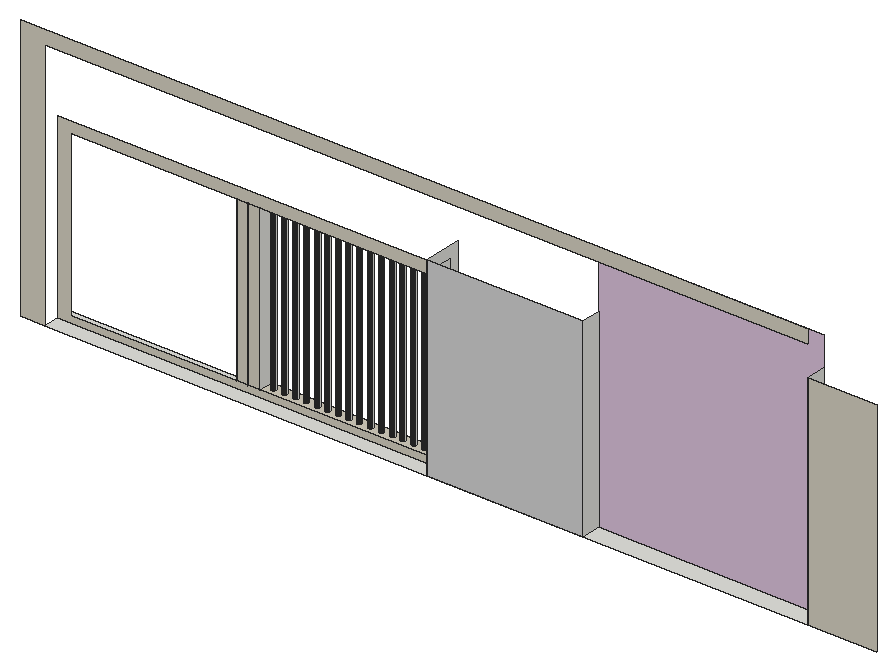
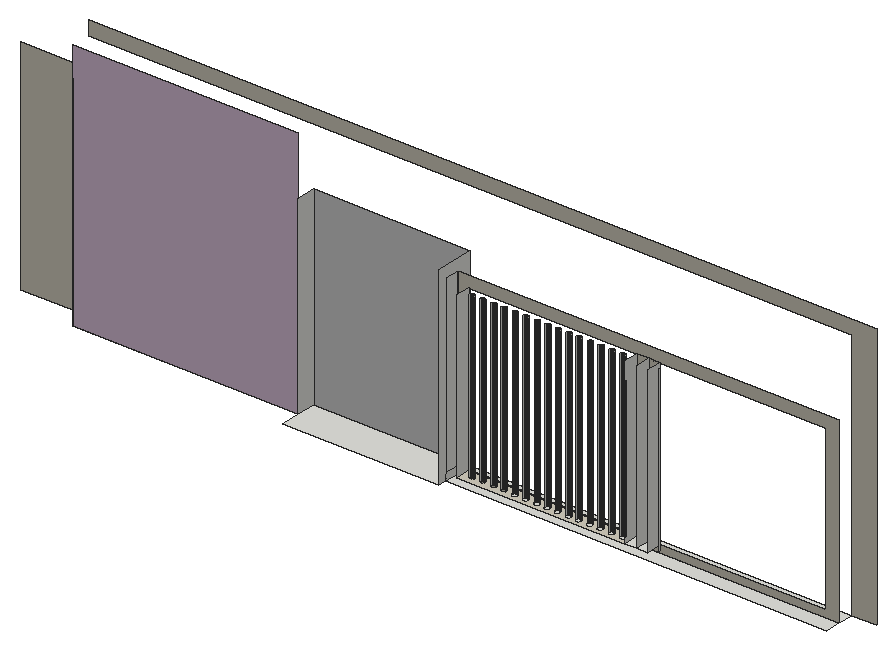
# SketchUp Ruby script. Lengths in inches.
U = 1.inch
M = Sketchup.active_model
def pt(a) = Geom::Point3d.new(a.map { |v| v * U })
def face(e, loops, mat)
  f = e.add_face(loops[0].map { |a| pt(a) })
  loops[1..].each { |l| e.add_face(l.map { |a| pt(a) }).erase! }
  f.material = f.back_material = mat if mat
  f
end
# faces: each face lists its corners as indices into pts; further lists are holes
def faces(e, pts, list, mat = nil) = list.each { |f| face(e, (f[0].is_a?(Array) ? f : [f]).map { |l| l.map { |i| pts[i] } }, mat) }
# xy, xz, yz: faces in a plane at the given z, y or x. An outline is a flat list of corners, or four numbers for a rectangle; further outlines are holes
def ring(l) = l.size == 4 ? [[l[0], l[1]], [l[2], l[1]], [l[2], l[3]], [l[0], l[3]]] : l.each_slice(2).to_a
def flat(e, list, mat, &to3) = list.each { |f| face(e, (f[0].is_a?(Array) ? f : [f]).map { |l| ring(l).map { |u, v| to3.(u, v) } }, mat) }
def xy(e, z, list, mat = nil) = flat(e, list, mat) { |x, y| [x, y, z] }
def xz(e, y, list, mat = nil) = flat(e, list, mat) { |x, z| [x, y, z] }
def yz(e, x, list, mat = nil) = flat(e, list, mat) { |y, z| [x, y, z] }
def lines(e, pts, list) = list.each { |a, b| e.add_line(pt(pts[a]), pt(pts[b])) }
# prism: a flat outline (further loops are holes) pulled along v
def prism(e, loops, v, mat = nil)
  f = face(e, loops, mat); d = Geom::Vector3d.new(v.map { |x| x * U })
  f.pushpull(f.normal.samedirection?(d) ? d.length : -d.length)
end
def box(e, o, s, mat = nil) = prism(e, [[o, [o[0] + s[0], o[1], o[2]], [o[0] + s[0], o[1] + s[1], o[2]], [o[0], o[1] + s[1], o[2]]]], [0, 0, s[2]], mat)
def at(x, y, z, deg = 0) = Geom::Transformation.translation(pt([x, y, z])) * Geom::Transformation.rotation(ORIGIN, Z_AXIS, deg.degrees)
def axes(o, x, y, z) = Geom::Transformation.new([*x, 0, *y, 0, *z, 0, *pt(o).to_a, 1])
def part(name) = M.definitions.add(name)
# library, detail: a bought-in or finely detailed component or shape, given as its bounding box
def library(name, o, s) = part(name).tap { |d| box(d.entities, o, s) }
def detail(e, o, s) = box(e.add_group.entities, o, s)
def put(e, d, t, mat = nil) = e.add_instance(d, t).tap { |i| i.material = mat if mat }
def group(e, t, mat = nil) = e.add_group.tap { |g| g.transformation = t; g.material = mat if mat }.entities
root = M.entities
M.materials.add("[0118_Thistle]").color = [216, 191, 216]
M.materials.add("[Cladding Siding White]").color = [207, 207, 207]
M.materials.add("[Formica Graystone]").color = [209, 204, 189]
xy(root,9,[[370.65,1.67,566.39,9.54],[566.39,1.67,646.62,21.38],[646.62,1.67,762.14,11.52],[370.65,9.54,566.39,17.41]])
xy(root,12.5,[[462.5,9.54,468.46,17.41],[468.46,9.54,474.42,17.41],[478.45,12.51,478.13,12.55,477.83,12.67,477.57,12.875,477.37,13.13,477.24,13.43,477.2,13.76,477.24,14.08,477.37,14.38,477.57,14.64,477.83,14.84,478.13,14.96,478.45,15.01,478.78,14.96,479.08,14.84,479.34,14.64,479.53,14.38,479.66,14.08,479.7,13.76,479.66,13.43,479.53,13.13,479.34,12.875,479.08,12.67,478.78,12.55],[484.01,12.51,483.69,12.55,483.39,12.67,483.13,12.875,482.93,13.13,482.81,13.43,482.76,13.76,482.81,14.08,482.93,14.38,483.13,14.64,483.39,14.84,483.69,14.96,484.01,15.01,484.34,14.96,484.64,14.84,484.9,14.64,485.1,14.38,485.22,14.08,485.26,13.76,485.22,13.43,485.1,13.13,484.9,12.875,484.64,12.67,484.34,12.55],[489.83,12.51,489.5,12.55,489.2,12.67,488.94,12.875,488.74,13.13,488.62,13.43,488.58,13.76,488.62,14.08,488.74,14.38,488.94,14.64,489.2,14.84,489.5,14.96,489.83,15.01,490.15,14.96,490.45,14.84,490.71,14.64,490.91,14.38,491.03,14.08,491.08,13.76,491.03,13.43,490.91,13.13,490.71,12.875,490.45,12.67,490.15,12.55],
  [495.14,12.51,494.82,12.55,494.51,12.67,494.26,12.875,494.06,13.13,493.93,13.43,493.89,13.76,493.93,14.08,494.06,14.38,494.26,14.64,494.51,14.84,494.82,14.96,495.14,15.01,495.46,14.96,495.76,14.84,496.02,14.64,496.22,14.38,496.35,14.08,496.39,13.76,496.35,13.43,496.22,13.13,496.02,12.875,495.76,12.67,495.46,12.55],[500.95,12.51,500.63,12.55,500.33,12.67,500.07,12.875,499.87,13.13,499.74,13.43,499.7,13.76,499.74,14.08,499.87,14.38,500.07,14.64,500.33,14.84,500.63,14.96,500.95,15.01,501.28,14.96,501.58,14.84,501.84,14.64,502.03,14.38,502.16,14.08,502.2,13.76,502.16,13.43,502.03,13.13,501.84,12.875,501.58,12.67,501.28,12.55],[506.08,12.51,505.75,12.55,505.45,12.67,505.19,12.875,504.99,13.13,504.87,13.43,504.83,13.76,504.87,14.08,504.99,14.38,505.19,14.64,505.45,14.84,505.75,14.96,506.08,15.01,506.4,14.96,506.7,14.84,506.96,14.64,507.16,14.38,507.28,14.08,507.33,13.76,507.28,13.43,507.16,13.13,506.96,12.875,506.7,12.67,506.4,12.55],[511.7,12.51,511.38,12.55,511.08,12.67,510.82,12.875,510.62,13.13,510.49,13.43,510.45,13.76,510.49,14.08,510.62,14.38,510.82,14.64,511.08,14.84,511.38,14.96,511.7,15.01,512.03,14.96,512.33,14.84,512.59,14.64,512.78,14.38,512.91,14.08,512.95,13.76,512.91,13.43,512.78,13.13,512.59,12.875,512.33,12.67,512.03,12.55],[517.01,12.51,516.69,12.55,516.39,12.67,516.13,12.875,515.93,13.13,515.81,13.43,515.76,13.76,515.81,14.08,515.93,14.38,516.13,14.64,516.39,14.84,516.69,14.96,517.01,15.01,517.34,14.96,517.64,14.84,517.9,14.64,518.1,14.38,518.22,14.08,518.26,13.76,518.22,13.43,518.1,13.13,517.9,12.875,517.64,12.67,517.34,12.55],
  [522.33,12.51,522,12.55,521.7,12.67,521.44,12.875,521.24,13.13,521.12,13.43,521.08,13.76,521.12,14.08,521.24,14.38,521.44,14.64,521.7,14.84,522,14.96,522.33,15.01,522.65,14.96,522.95,14.84,523.21,14.64,523.41,14.38,523.53,14.08,523.58,13.76,523.53,13.43,523.41,13.13,523.21,12.875,522.95,12.67,522.65,12.55],[528.2,12.51,527.88,12.55,527.58,12.67,527.32,12.875,527.12,13.13,526.99,13.43,526.95,13.76,526.99,14.08,527.12,14.38,527.32,14.64,527.58,14.84,527.88,14.96,528.2,15.01,528.53,14.96,528.83,14.84,529.09,14.64,529.28,14.38,529.41,14.08,529.45,13.76,529.41,13.43,529.28,13.13,529.09,12.875,528.83,12.67,528.53,12.55],[533.7,12.51,533.38,12.55,533.08,12.67,532.82,12.875,532.62,13.13,532.49,13.43,532.45,13.76,532.49,14.08,532.62,14.38,532.82,14.64,533.08,14.84,533.38,14.96,533.7,15.01,534.03,14.96,534.33,14.84,534.59,14.64,534.78,14.38,534.91,14.08,534.95,13.76,534.91,13.43,534.78,13.13,534.59,12.875,534.33,12.67,534.03,12.55]])
xy(root,12.5,[[[474.42,9.54,560.77,17.41],[478.45,12.51,478.13,12.55,477.83,12.67,477.57,12.875,477.37,13.13,477.24,13.43,477.2,13.76,477.24,14.08,477.37,14.38,477.57,14.64,477.83,14.84,478.13,14.96,478.45,15.01,478.78,14.96,479.08,14.84,479.34,14.64,479.53,14.38,479.66,14.08,479.7,13.76,479.66,13.43,479.53,13.13,479.34,12.875,479.08,12.67,478.78,12.55],[555.89,12.51,555.57,12.55,555.26,12.67,555.01,12.875,554.81,13.13,554.68,13.43,554.64,13.76,554.68,14.08,554.81,14.38,555.01,14.64,555.26,14.84,555.57,14.96,555.89,15.01,556.21,14.96,556.51,14.84,556.77,14.64,556.97,14.38,557.1,14.08,557.14,13.76,557.1,13.43,556.97,13.13,556.77,12.875,556.51,12.67,556.21,12.55],[484.01,12.51,483.69,12.55,483.39,12.67,483.13,12.875,482.93,13.13,482.81,13.43,482.76,13.76,482.81,14.08,482.93,14.38,483.13,14.64,483.39,14.84,483.69,14.96,484.01,15.01,484.34,14.96,484.64,14.84,484.9,14.64,485.1,14.38,485.22,14.08,485.26,13.76,485.22,13.43,485.1,13.13,484.9,12.875,484.64,12.67,484.34,12.55],[550.39,12.51,550.07,12.55,549.76,12.67,549.51,12.875,549.31,13.13,549.18,13.43,549.14,13.76,549.18,14.08,549.31,14.38,549.51,14.64,549.76,14.84,550.07,14.96,550.39,15.01,550.71,14.96,551.01,14.84,551.27,14.64,551.47,14.38,551.6,14.08,551.64,13.76,551.6,13.43,551.47,13.13,551.27,12.875,551.01,12.67,550.71,12.55],[489.83,12.51,489.5,12.55,489.2,12.67,488.94,12.875,488.74,13.13,488.62,13.43,488.58,13.76,488.62,14.08,488.74,14.38,488.94,14.64,489.2,14.84,489.5,14.96,489.83,15.01,490.15,14.96,490.45,14.84,490.71,14.64,490.91,14.38,491.03,14.08,491.08,13.76,491.03,13.43,490.91,13.13,490.71,12.875,490.45,12.67,490.15,12.55],[544.76,12.51,544.44,12.55,544.14,12.67,543.88,12.875,543.68,13.13,543.56,13.43,543.51,13.76,543.56,14.08,543.68,14.38,543.88,14.64,544.14,14.84,544.44,14.96,544.76,15.01,545.09,14.96,545.39,14.84,545.65,14.64,545.85,14.38,545.97,14.08,546.01,13.76,545.97,13.43,545.85,13.13,545.65,12.875,545.39,12.67,545.09,12.55],[495.14,12.51,494.82,12.55,494.51,12.67,494.26,12.875,494.06,13.13,493.93,13.43,493.89,13.76,493.93,14.08,494.06,14.38,494.26,14.64,494.51,14.84,494.82,14.96,495.14,15.01,495.46,14.96,495.76,14.84,496.02,14.64,496.22,14.38,496.35,14.08,496.39,13.76,496.35,13.43,496.22,13.13,496.02,12.875,495.76,12.67,495.46,12.55],[539.51,12.51,539.19,12.55,538.89,12.67,538.63,12.875,538.43,13.13,538.31,13.43,538.26,13.76,538.31,14.08,538.43,14.38,538.63,14.64,538.89,14.84,539.19,14.96,539.51,15.01,539.84,14.96,540.14,14.84,540.4,14.64,540.6,14.38,540.72,14.08,540.76,13.76,540.72,13.43,540.6,13.13,540.4,12.875,540.14,12.67,539.84,12.55],[500.95,12.51,500.63,12.55,500.33,12.67,500.07,12.875,499.87,13.13,499.74,13.43,499.7,13.76,499.74,14.08,499.87,14.38,500.07,14.64,500.33,14.84,500.63,14.96,500.95,15.01,501.28,14.96,501.58,14.84,501.84,14.64,502.03,14.38,502.16,14.08,502.2,13.76,502.16,13.43,502.03,13.13,501.84,12.875,501.58,12.67,501.28,12.55],[533.7,12.51,533.38,12.55,533.08,12.67,532.82,12.875,532.62,13.13,532.49,13.43,532.45,13.76,532.49,14.08,532.62,14.38,532.82,14.64,533.08,14.84,533.38,14.96,533.7,15.01,534.03,14.96,534.33,14.84,534.59,14.64,534.78,14.38,534.91,14.08,534.95,13.76,534.91,13.43,534.78,13.13,534.59,12.875,534.33,12.67,534.03,12.55],[506.08,12.51,505.75,12.55,505.45,12.67,505.19,12.875,504.99,13.13,504.87,13.43,504.83,13.76,504.87,14.08,504.99,14.38,505.19,14.64,505.45,14.84,505.75,14.96,506.08,15.01,506.4,14.96,506.7,14.84,506.96,14.64,507.16,14.38,507.28,14.08,507.33,13.76,507.28,13.43,507.16,13.13,506.96,12.875,506.7,12.67,506.4,12.55],[528.2,12.51,527.88,12.55,527.58,12.67,527.32,12.875,527.12,13.13,526.99,13.43,526.95,13.76,526.99,14.08,527.12,14.38,527.32,14.64,527.58,14.84,527.88,14.96,528.2,15.01,528.53,14.96,528.83,14.84,529.09,14.64,529.28,14.38,529.41,14.08,529.45,13.76,529.41,13.43,529.28,13.13,529.09,12.875,528.83,12.67,528.53,12.55],[511.7,12.51,511.38,12.55,511.08,12.67,510.82,12.875,510.62,13.13,510.49,13.43,510.45,13.76,510.49,14.08,510.62,14.38,510.82,14.64,511.08,14.84,511.38,14.96,511.7,15.01,512.03,14.96,512.33,14.84,512.59,14.64,512.78,14.38,512.91,14.08,512.95,13.76,512.91,13.43,512.78,13.13,512.59,12.875,512.33,12.67,512.03,12.55],[517.01,12.51,516.69,12.55,516.39,12.67,516.13,12.875,515.93,13.13,515.81,13.43,515.76,13.76,515.81,14.08,515.93,14.38,516.13,14.64,516.39,14.84,516.69,14.96,517.01,15.01,517.34,14.96,517.64,14.84,517.9,14.64,518.1,14.38,518.22,14.08,518.26,13.76,518.22,13.43,518.1,13.13,517.9,12.875,517.64,12.67,517.34,12.55],[522.33,12.51,522,12.55,521.7,12.67,521.44,12.875,521.24,13.13,521.12,13.43,521.08,13.76,521.12,14.08,521.24,14.38,521.44,14.64,521.7,14.84,522,14.96,522.33,15.01,522.65,14.96,522.95,14.84,523.21,14.64,523.41,14.38,523.53,14.08,523.58,13.76,523.53,13.43,523.41,13.13,523.21,12.875,522.95,12.67,522.65,12.55]]],"[Formica Graystone]")
xz(root,1.67,[[566.39,9,646.62,108]],"[Cladding Siding White]")
xz(root,1.67,[[357.9375,9,370.65,9,370.65,138.11,762.14,138.11,762.14,145.125,357.9375,145.125],[762.14,9,797.12,122.6875]],"[Formica Graystone]")
xz(root,9.54,[[[370.65,9,566.39,102.25],[377.34,12.5,560.77,96.37]],[462.5,12.5,468.46,96.37],[468.46,12.5,474.42,96.37]],"[Formica Graystone]")
xz(root,11.52,[[646.62,9,762.14,138.11]],"[0118_Thistle]")
yz(root,462.5,[[9.54,12.5,17.41,96.37]])
yz(root,468.46,[[9.54,12.5,17.41,96.37]])
yz(root,474.42,[[9.54,12.5,17.41,96.37]])
yz(root,560.77,[[9.54,12.5,17.41,96.37]])
yz(root,566.39,[[1.67,9,1.67,108,21.38,108,21.38,9,17.41,9,17.41,102.25,9.54,102.25,9.54,9],[9.54,9,17.41,12.5],[9.54,12.5,17.41,102.25]])
yz(root,646.62,[[1.67,9,11.52,108]])
yz(root,762.14,[[1.67,9,11.52,122.6875]])
p = [[477.83,12.67,12.5],[478.13,12.55,12.5],[478.13,12.55,96.37],[477.83,12.67,96.37],[478.45,12.51,12.5],[478.45,12.51,96.37],
  [478.78,12.55,12.5],[478.78,12.55,96.37],[479.08,12.67,12.5],[479.08,12.67,96.37],[483.39,12.67,12.5],[483.69,12.55,12.5],
  [483.69,12.55,96.37],[483.39,12.67,96.37],[484.01,12.51,12.5],[484.01,12.51,96.37],[484.34,12.55,12.5],[484.34,12.55,96.37],
  [484.64,12.67,12.5],[484.64,12.67,96.37],[489.2,12.67,12.5],[489.5,12.55,12.5],[489.5,12.55,96.37],[489.2,12.67,96.37],
  [489.83,12.51,12.5],[489.83,12.51,96.37],[490.15,12.55,12.5],[490.15,12.55,96.37],[490.45,12.67,12.5],[490.45,12.67,96.37],
  [494.51,12.67,12.5],[494.82,12.55,12.5],[494.82,12.55,96.37],[494.51,12.67,96.37],[495.14,12.51,12.5],[495.14,12.51,96.37],
  [495.46,12.55,12.5],[495.46,12.55,96.37],[495.76,12.67,12.5],[495.76,12.67,96.37],[500.33,12.67,12.5],[500.63,12.55,12.5],
  [500.63,12.55,96.37],[500.33,12.67,96.37],[500.95,12.51,12.5],[500.95,12.51,96.37],[501.28,12.55,12.5],[501.28,12.55,96.37],
  [501.58,12.67,12.5],[501.58,12.67,96.37],[505.45,12.67,12.5],[505.75,12.55,12.5],[505.75,12.55,96.37],[505.45,12.67,96.37],
  [506.08,12.51,12.5],[506.08,12.51,96.37],[506.4,12.55,12.5],[506.4,12.55,96.37],[506.7,12.67,12.5],[506.7,12.67,96.37],
  [511.08,12.67,12.5],[511.38,12.55,12.5],[511.38,12.55,96.37],[511.08,12.67,96.37],[511.7,12.51,12.5],[511.7,12.51,96.37],
  [512.03,12.55,12.5],[512.03,12.55,96.37],[512.33,12.67,12.5],[512.33,12.67,96.37],[516.39,12.67,12.5],[516.69,12.55,12.5],
  [516.69,12.55,96.37],[516.39,12.67,96.37],[517.01,12.51,12.5],[517.01,12.51,96.37],[517.34,12.55,12.5],[517.34,12.55,96.37],
  [517.64,12.67,12.5],[517.64,12.67,96.37],[521.7,12.67,12.5],[522,12.55,12.5],[522,12.55,96.37],[521.7,12.67,96.37],
  [522.33,12.51,12.5],[522.33,12.51,96.37],[522.65,12.55,12.5],[522.65,12.55,96.37],[522.95,12.67,12.5],[522.95,12.67,96.37],
  [527.58,12.67,12.5],[527.88,12.55,12.5],[527.88,12.55,96.37],[527.58,12.67,96.37],[528.2,12.51,12.5],[528.2,12.51,96.37],
  [528.53,12.55,12.5],[528.53,12.55,96.37],[528.83,12.67,12.5],[528.83,12.67,96.37],[533.08,12.67,12.5],[533.38,12.55,12.5],
  [533.38,12.55,96.37],[533.08,12.67,96.37],[533.7,12.51,12.5],[533.7,12.51,96.37],[534.03,12.55,12.5],[534.03,12.55,96.37],
  [534.33,12.67,12.5],[534.33,12.67,96.37],[538.89,12.67,12.5],[539.19,12.55,12.5],[539.19,12.55,96.37],[538.89,12.67,96.37],
  [539.51,12.51,12.5],[539.51,12.51,96.37],[539.84,12.55,12.5],[539.84,12.55,96.37],[540.14,12.67,12.5],[540.14,12.67,96.37],
  [544.14,12.67,12.5],[544.44,12.55,12.5],[544.44,12.55,96.37],[544.14,12.67,96.37],[544.76,12.51,12.5],[544.76,12.51,96.37],
  [545.09,12.55,12.5],[545.09,12.55,96.37],[545.39,12.67,12.5],[545.39,12.67,96.37],[549.76,12.67,12.5],[550.07,12.55,12.5],
  [550.07,12.55,96.37],[549.76,12.67,96.37],[550.39,12.51,12.5],[550.39,12.51,96.37],[550.71,12.55,12.5],[550.71,12.55,96.37],
  [551.01,12.67,12.5],[551.01,12.67,96.37],[555.26,12.67,12.5],[555.57,12.55,12.5],[555.57,12.55,96.37],[555.26,12.67,96.37],
  [555.89,12.51,12.5],[555.89,12.51,96.37],[556.21,12.55,12.5],[556.21,12.55,96.37],[556.51,12.67,12.5],[556.51,12.67,96.37],
  [477.57,12.875,12.5],[477.57,12.875,96.37],[479.34,12.875,12.5],[479.34,12.875,96.37],[483.13,12.875,12.5],[483.13,12.875,96.37],
  [484.9,12.875,12.5],[484.9,12.875,96.37],[488.94,12.875,12.5],[488.94,12.875,96.37],[490.71,12.875,12.5],[490.71,12.875,96.37],
  [494.26,12.875,12.5],[494.26,12.875,96.37],[496.02,12.875,12.5],[496.02,12.875,96.37],[500.07,12.875,12.5],[500.07,12.875,96.37],
  [501.84,12.875,12.5],[501.84,12.875,96.37],[505.19,12.875,12.5],[505.19,12.875,96.37],[506.96,12.875,12.5],[506.96,12.875,96.37],
  [510.82,12.875,12.5],[510.82,12.875,96.37],[512.59,12.875,12.5],[512.59,12.875,96.37],[516.13,12.875,12.5],[516.13,12.875,96.37],
  [517.9,12.875,12.5],[517.9,12.875,96.37],[521.44,12.875,12.5],[521.44,12.875,96.37],[523.21,12.875,12.5],[523.21,12.875,96.37],
  [527.32,12.875,12.5],[527.32,12.875,96.37],[529.09,12.875,12.5],[529.09,12.875,96.37],[532.82,12.875,12.5],[532.82,12.875,96.37],
  [534.59,12.875,12.5],[534.59,12.875,96.37],[538.63,12.875,12.5],[538.63,12.875,96.37],[540.4,12.875,12.5],[540.4,12.875,96.37],
  [543.88,12.875,12.5],[543.88,12.875,96.37],[545.65,12.875,12.5],[545.65,12.875,96.37],[549.51,12.875,12.5],[549.51,12.875,96.37],
  [551.27,12.875,12.5],[551.27,12.875,96.37],[555.01,12.875,12.5],[555.01,12.875,96.37],[556.77,12.875,12.5],[556.77,12.875,96.37],
  [477.37,13.13,12.5],[477.37,13.13,96.37],[479.53,13.13,12.5],[479.53,13.13,96.37],[482.93,13.13,12.5],[482.93,13.13,96.37],
  [485.1,13.13,12.5],[485.1,13.13,96.37],[488.74,13.13,12.5],[488.74,13.13,96.37],[490.91,13.13,12.5],[490.91,13.13,96.37],
  [494.06,13.13,12.5],[494.06,13.13,96.37],[496.22,13.13,12.5],[496.22,13.13,96.37],[499.87,13.13,12.5],[499.87,13.13,96.37],
  [502.03,13.13,12.5],[502.03,13.13,96.37],[504.99,13.13,12.5],[504.99,13.13,96.37],[507.16,13.13,12.5],[507.16,13.13,96.37],
  [510.62,13.13,12.5],[510.62,13.13,96.37],[512.78,13.13,12.5],[512.78,13.13,96.37],[515.93,13.13,12.5],[515.93,13.13,96.37],
  [518.1,13.13,12.5],[518.1,13.13,96.37],[521.24,13.13,12.5],[521.24,13.13,96.37],[523.41,13.13,12.5],[523.41,13.13,96.37],
  [527.12,13.13,12.5],[527.12,13.13,96.37],[529.28,13.13,12.5],[529.28,13.13,96.37],[532.62,13.13,12.5],[532.62,13.13,96.37],
  [534.78,13.13,12.5],[534.78,13.13,96.37],[538.43,13.13,12.5],[538.43,13.13,96.37],[540.6,13.13,12.5],[540.6,13.13,96.37],
  [543.68,13.13,12.5],[543.68,13.13,96.37],[545.85,13.13,12.5],[545.85,13.13,96.37],[549.31,13.13,12.5],[549.31,13.13,96.37],
  [551.47,13.13,12.5],[551.47,13.13,96.37],[554.81,13.13,12.5],[554.81,13.13,96.37],[556.97,13.13,12.5],[556.97,13.13,96.37],
  [477.24,13.43,12.5],[477.24,13.43,96.37],[479.66,13.43,12.5],[479.66,13.43,96.37],[482.81,13.43,12.5],[482.81,13.43,96.37],
  [485.22,13.43,12.5],[485.22,13.43,96.37],[488.62,13.43,12.5],[488.62,13.43,96.37],[491.03,13.43,12.5],[491.03,13.43,96.37],
  [493.93,13.43,12.5],[493.93,13.43,96.37],[496.35,13.43,12.5],[496.35,13.43,96.37],[499.74,13.43,12.5],[499.74,13.43,96.37],
  [502.16,13.43,12.5],[502.16,13.43,96.37],[504.87,13.43,12.5],[504.87,13.43,96.37],[507.28,13.43,12.5],[507.28,13.43,96.37],
  [510.49,13.43,12.5],[510.49,13.43,96.37],[512.91,13.43,12.5],[512.91,13.43,96.37],[515.81,13.43,12.5],[515.81,13.43,96.37],
  [518.22,13.43,12.5],[518.22,13.43,96.37],[521.12,13.43,12.5],[521.12,13.43,96.37],[523.53,13.43,12.5],[523.53,13.43,96.37],
  [526.99,13.43,12.5],[526.99,13.43,96.37],[529.41,13.43,12.5],[529.41,13.43,96.37],[532.49,13.43,12.5],[532.49,13.43,96.37],
  [534.91,13.43,12.5],[534.91,13.43,96.37],[538.31,13.43,12.5],[538.31,13.43,96.37],[540.72,13.43,12.5],[540.72,13.43,96.37],
  [543.56,13.43,12.5],[543.56,13.43,96.37],[545.97,13.43,12.5],[545.97,13.43,96.37],[549.18,13.43,12.5],[549.18,13.43,96.37],
  [551.6,13.43,12.5],[551.6,13.43,96.37],[554.68,13.43,12.5],[554.68,13.43,96.37],[557.1,13.43,12.5],[557.1,13.43,96.37],
  [459.85,13.43,12.5],[459.89,13.76,12.5],[459.89,13.76,96.37],[459.85,13.43,96.37],[477.2,13.76,12.5],[477.2,13.76,96.37],
  [479.7,13.76,12.5],[479.7,13.76,96.37],[482.76,13.76,12.5],[482.76,13.76,96.37],[485.26,13.76,12.5],[485.26,13.76,96.37],
  [488.58,13.76,12.5],[488.58,13.76,96.37],[491.08,13.76,12.5],[491.08,13.76,96.37],[493.89,13.76,12.5],[493.89,13.76,96.37],
  [496.39,13.76,12.5],[496.39,13.76,96.37],[499.7,13.76,12.5],[499.7,13.76,96.37],[502.2,13.76,12.5],[502.2,13.76,96.37],
  [504.83,13.76,12.5],[504.83,13.76,96.37],[507.33,13.76,12.5],[507.33,13.76,96.37],[510.45,13.76,12.5],[510.45,13.76,96.37],
  [512.95,13.76,12.5],[512.95,13.76,96.37],[515.76,13.76,12.5],[515.76,13.76,96.37],[518.26,13.76,12.5],[518.26,13.76,96.37],
  [521.08,13.76,12.5],[521.08,13.76,96.37],[523.58,13.76,12.5],[523.58,13.76,96.37],[526.95,13.76,12.5],[526.95,13.76,96.37],
  [529.45,13.76,12.5],[529.45,13.76,96.37],[532.45,13.76,12.5],[532.45,13.76,96.37],[534.95,13.76,12.5],[534.95,13.76,96.37],
  [538.26,13.76,12.5],[538.26,13.76,96.37],[540.76,13.76,12.5],[540.76,13.76,96.37],[543.51,13.76,12.5],[543.51,13.76,96.37],
  [546.01,13.76,12.5],[546.01,13.76,96.37],[549.14,13.76,12.5],[549.14,13.76,96.37],[551.64,13.76,12.5],[551.64,13.76,96.37],
  [554.64,13.76,12.5],[554.64,13.76,96.37],[557.14,13.76,12.5],[557.14,13.76,96.37]]
faces(root,p,[[0,1,2,3],[1,4,5,2],[4,6,7,5],[6,8,9,7],[10,11,12,13],[11,14,15,12],[14,16,17,15],[16,18,19,17],
  [20,21,22,23],[21,24,25,22],[24,26,27,25],[26,28,29,27],[30,31,32,33],[31,34,35,32],[34,36,37,35],[36,38,39,37],
  [40,41,42,43],[41,44,45,42],[44,46,47,45],[46,48,49,47],[50,51,52,53],[51,54,55,52],[54,56,57,55],[56,58,59,57],
  [60,61,62,63],[61,64,65,62],[64,66,67,65],[66,68,69,67],[70,71,72,73],[71,74,75,72],[74,76,77,75],[76,78,79,77],
  [80,81,82,83],[81,84,85,82],[84,86,87,85],[86,88,89,87],[90,91,92,93],[91,94,95,92],[94,96,97,95],[96,98,99,97],
  [100,101,102,103],[101,104,105,102],[104,106,107,105],[106,108,109,107],[110,111,112,113],[111,114,115,112],[114,116,117,115],[116,118,119,117],
  [120,121,122,123],[121,124,125,122],[124,126,127,125],[126,128,129,127],[130,131,132,133],[131,134,135,132],[134,136,137,135],[136,138,139,137],
  [140,141,142,143],[141,144,145,142],[144,146,147,145],[146,148,149,147],[150,0,3,151],[8,152,153,9],[154,10,13,155],[18,156,157,19],
  [158,20,23,159],[28,160,161,29],[162,30,33,163],[38,164,165,39],[166,40,43,167],[48,168,169,49],[170,50,53,171],[58,172,173,59],
  [174,60,63,175],[68,176,177,69],[178,70,73,179],[78,180,181,79],[182,80,83,183],[88,184,185,89],[186,90,93,187],[98,188,189,99],
  [190,100,103,191],[108,192,193,109],[194,110,113,195],[118,196,197,119],[198,120,123,199],[128,200,201,129],[202,130,133,203],[138,204,205,139],
  [206,140,143,207],[148,208,209,149],[210,150,151,211],[152,212,213,153],[214,154,155,215],[156,216,217,157],[218,158,159,219],[160,220,221,161],
  [222,162,163,223],[164,224,225,165],[226,166,167,227],[168,228,229,169],[230,170,171,231],[172,232,233,173],[234,174,175,235],[176,236,237,177],
  [238,178,179,239],[180,240,241,181],[242,182,183,243],[184,244,245,185],[246,186,187,247],[188,248,249,189],[250,190,191,251],[192,252,253,193],
  [254,194,195,255],[196,256,257,197],[258,198,199,259],[200,260,261,201],[262,202,203,263],[204,264,265,205],[266,206,207,267],[208,268,269,209],
  [270,210,211,271],[212,272,273,213],[274,214,215,275],[216,276,277,217],[278,218,219,279],[220,280,281,221],[282,222,223,283],[224,284,285,225],
  [286,226,227,287],[228,288,289,229],[290,230,231,291],[232,292,293,233],[294,234,235,295],[236,296,297,237],[298,238,239,299],[240,300,301,241],
  [302,242,243,303],[244,304,305,245],[306,246,247,307],[248,308,309,249],[310,250,251,311],[252,312,313,253],[314,254,255,315],[256,316,317,257],
  [318,258,259,319],[260,320,321,261],[322,262,263,323],[264,324,325,265],[326,266,267,327],[268,328,329,269],[330,331,332,333],[334,270,271,335],
  [272,336,337,273],[338,274,275,339],[276,340,341,277],[342,278,279,343],[280,344,345,281],[346,282,283,347],[284,348,349,285],[350,286,287,351],
  [288,352,353,289],[354,290,291,355],[292,356,357,293],[358,294,295,359],[296,360,361,297],[362,298,299,363],[300,364,365,301],[366,302,303,367],
  [304,368,369,305],[370,306,307,371],[308,372,373,309],[374,310,311,375],[312,376,377,313],[378,314,315,379],[316,380,381,317],[382,318,319,383],
  [320,384,385,321],[386,322,323,387],[324,388,389,325],[390,326,327,391],[328,392,393,329]])
